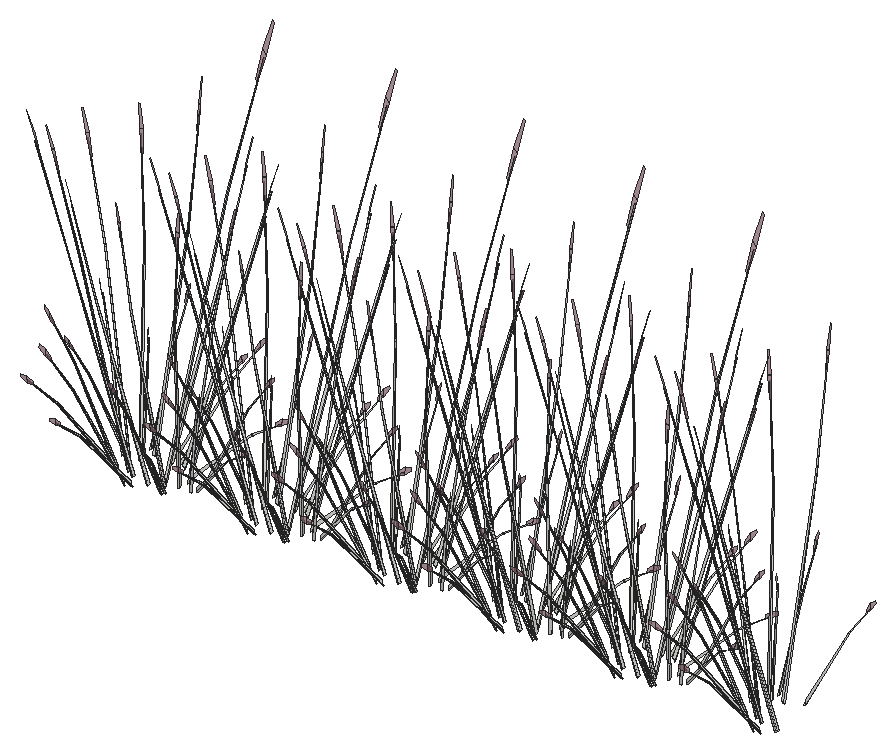
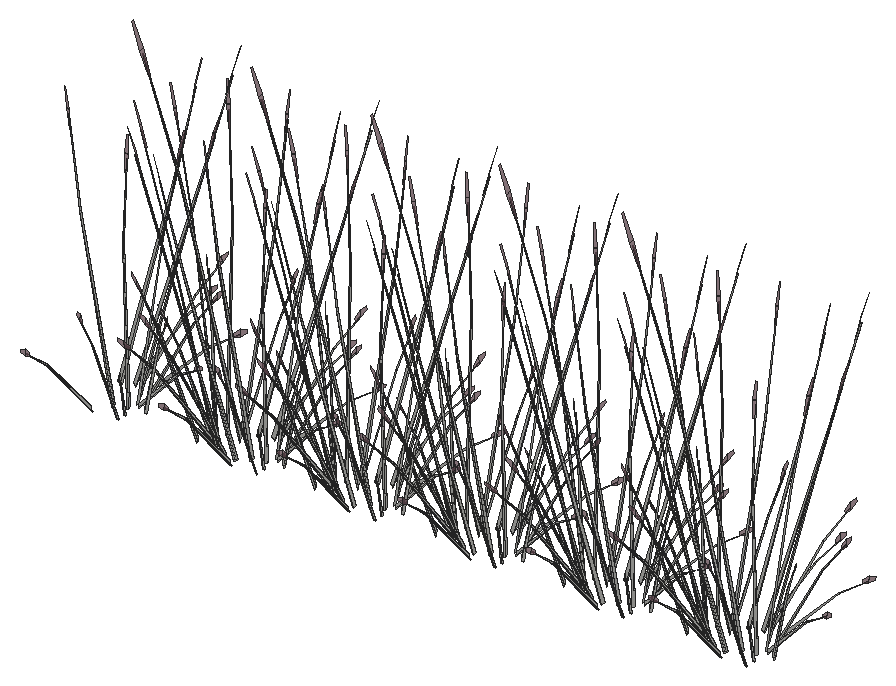
# SketchUp Ruby script. Lengths in inches.
U = 1.inch
M = Sketchup.active_model
def pt(a) = Geom::Point3d.new(a.map { |v| v * U })
def face(e, loops, mat)
  f = e.add_face(loops[0].map { |a| pt(a) })
  loops[1..].each { |l| e.add_face(l.map { |a| pt(a) }).erase! }
  f.material = f.back_material = mat if mat
  f
end
# faces: each face lists its corners as indices into pts; further lists are holes
def faces(e, pts, list, mat = nil) = list.each { |f| face(e, (f[0].is_a?(Array) ? f : [f]).map { |l| l.map { |i| pts[i] } }, mat) }
# xy, xz, yz: faces in a plane at the given z, y or x. An outline is a flat list of corners, or four numbers for a rectangle; further outlines are holes
def ring(l) = l.size == 4 ? [[l[0], l[1]], [l[2], l[1]], [l[2], l[3]], [l[0], l[3]]] : l.each_slice(2).to_a
def flat(e, list, mat, &to3) = list.each { |f| face(e, (f[0].is_a?(Array) ? f : [f]).map { |l| ring(l).map { |u, v| to3.(u, v) } }, mat) }
def xy(e, z, list, mat = nil) = flat(e, list, mat) { |x, y| [x, y, z] }
def xz(e, y, list, mat = nil) = flat(e, list, mat) { |x, z| [x, y, z] }
def yz(e, x, list, mat = nil) = flat(e, list, mat) { |y, z| [x, y, z] }
def lines(e, pts, list) = list.each { |a, b| e.add_line(pt(pts[a]), pt(pts[b])) }
# prism: a flat outline (further loops are holes) pulled along v
def prism(e, loops, v, mat = nil)
  f = face(e, loops, mat); d = Geom::Vector3d.new(v.map { |x| x * U })
  f.pushpull(f.normal.samedirection?(d) ? d.length : -d.length)
end
def box(e, o, s, mat = nil) = prism(e, [[o, [o[0] + s[0], o[1], o[2]], [o[0] + s[0], o[1] + s[1], o[2]], [o[0], o[1] + s[1], o[2]]]], [0, 0, s[2]], mat)
def at(x, y, z, deg = 0) = Geom::Transformation.translation(pt([x, y, z])) * Geom::Transformation.rotation(ORIGIN, Z_AXIS, deg.degrees)
def axes(o, x, y, z) = Geom::Transformation.new([*x, 0, *y, 0, *z, 0, *pt(o).to_a, 1])
def part(name) = M.definitions.add(name)
# library, detail: a bought-in or finely detailed component or shape, given as its bounding box
def library(name, o, s) = part(name).tap { |d| box(d.entities, o, s) }
def detail(e, o, s) = box(e.add_group.entities, o, s)
def put(e, d, t, mat = nil) = e.add_instance(d, t).tap { |i| i.material = mat if mat }
def group(e, t, mat = nil) = e.add_group.tap { |g| g.transformation = t; g.material = mat if mat }.entities
root = M.entities
M.materials.add("LightPink_Translucent").color = [144, 107, 117]
M.materials["LightPink_Translucent"].alpha = 0.75
c1 = part("blade")
p = [[2.15,0.21,22],[0,0.17,0],[0.09,0.45,0],[2.18,0.31,22],[2.29,0.31,22],[0.38,0.45,0],
  [2.48,0.24,33],[2.49,0.24,33],[2.48,0.22,33]]
faces(c1.entities,p,[[0,1,2,3],[4,5,2,3],[6,3,4,7],[8,0,3,6]])
c2 = part("seeds")
p = [[0.3,-0.1,1.38],[-0.01,-0.03,1.59],[-0.01,-0.03,0.03],[0.14,-0.07,-0.07],[0.29,-0.03,3],[0.15,0.01,3.11]]
faces(c2.entities,p,[[0,1,2,3],[1,0,4,5]],"LightPink_Translucent")
c3 = part("blade with seeds")
put(c3.entities,c1,at(0,0,0))
put(c3.entities,c2,axes([2.4,0.25,30.99],[1.5799,-0.05474,1.17369],[-0.12525,1.92788,0.29478],[-0.07173,-0.02425,1.56792]))
put(root,c3,axes([241.68,53.5625,259.72],[-0.12407,0.07933,1.74944],[0.01055,0.57963,-0.27667],[-0.2844,0.07538,0.14031]))
put(root,c3,axes([240.3,54.15,259.71],[0.09697,0.01639,1.77383],[0.29997,0.53988,-0.16761],[-0.1985,0.1417,0.31391]))
put(root,c3,axes([242.27,51.15,259.71],[0.05633,0.06098,1.77383],[-0.27155,0.54815,-0.16761],[-0.27501,0.00397,0.31391]))
put(root,c3,axes([242.9,50.78,259.72],[-0.16348,-0.00431,1.74944],[-0.52047,0.43131,-0.27667],[-0.2777,-0.08813,0.14031]))
put(root,c3,axes([242.48,53.01,260.03],[0.38229,0.5533,-0.1216],[-0.6785,0.2719,-0.67495],[-0.28593,0.073,1.02557]))
put(root,c3,axes([243.34,51.86,260.03],[-0.04068,0.62141,-0.1216],[-0.77029,-0.01698,-0.67495],[-0.29667,-0.04317,1.02557]))
put(root,c3,axes([241.7,55.73,259.72],[-0.01889,0.12092,1.74944],[0.53598,0.42065,-0.27667],[-0.14032,0.19892,0.14031]))
put(root,c3,axes([244.84,50.95,260.43],[-0.50709,0.58578,-0.13619],[-0.73436,-0.33748,-0.75594],[-0.25527,-0.1655,1.14864]))
put(root,c3,axes([242.51,54.33,260.03],[0.70283,0.33692,-0.1216],[-0.40491,0.48793,-0.67495],[-0.19857,0.16961,1.02557]))
put(root,c3,axes([244.65,49.56,259.71],[-0.01417,0.07324,1.77383],[-0.6991,0.2658,-0.16761],[-0.20573,-0.13587,0.31391]))
put(root,c3,axes([241.64,56.97,259.71],[0.0862,-0.03689,1.77383],[0.71245,0.24539,-0.16761],[-0.01674,0.20431,0.31391]))
put(root,c3,axes([245.44,49.84,259.72],[-0.11621,-0.08567,1.74944],[-0.77555,0.05431,-0.27667],[-0.12378,-0.20491,0.14031]))
put(root,c3,axes([243.42,55.45,260.4],[0.83505,0.03027,-0.13498],[-0.02282,0.57322,-0.74919],[-0.05801,0.22077,1.13838]))
put(root,c3,axes([246.62,51.16,260.03],[-0.74352,0.28449,-0.1216],[-0.36538,-0.50492,-0.67495],[-0.0981,-0.21277,1.02557]))
put(root,c3,axes([244.79,57.22,259.72],[0.09631,0.0984,1.74944],[0.77725,0.03866,-0.27667],[0.07816,0.217,0.14031]))
put(root,c3,axes([244.96,56.09,260.03],[0.74352,-0.28449,-0.1216],[0.36538,0.50492,-0.67495],[0.0981,0.21277,1.02557]))
put(root,c3,axes([248.76,50.45,259.71],[-0.07716,0.04667,1.77383],[-0.75601,-0.15746,-0.16761],[-0.02737,-0.20368,0.31391]))
put(root,c3,axes([248.17,51.8,260.03],[-0.83505,-0.03027,-0.1216],[0.02282,-0.57322,-0.67495],[0.05801,-0.22077,1.02557]))
put(root,c3,axes([247.24,52.99,259.47],[-0.65655,-0.31748,1.38283],[0.69326,-0.49431,0.59665],[0.21183,0.29789,1.33663]))
put(root,c3,axes([246.14,56.51,259.71],[0.00225,-0.07398,1.77383],[0.65113,-0.32638,-0.16761],[0.22617,0.1165,0.31391]))
put(root,c3,axes([248.93,50.89,259.72],[-0.00733,-0.12161,1.74944],[-0.61946,-0.35147,-0.27667],[0.09577,-0.21306,0.14031]))
put(root,c3,axes([246.73,56.07,260.03],[0.45276,-0.52302,-0.1216],[0.65568,0.30132,-0.67495],[0.22792,0.14777,1.02557]))
put(root,c3,axes([249.08,52.93,260.03],[-0.70283,-0.33692,-0.1216],[0.40491,-0.48793,-0.67495],[0.19857,-0.16961,1.02557]))
put(root,c3,axes([257.75,53.5625,259.72],[-0.12407,0.07933,1.74944],[0.01055,0.57963,-0.27667],[-0.2844,0.07538,0.14031]))
put(root,c3,axes([256.37,54.15,259.71],[0.09697,0.01639,1.77383],[0.29997,0.53988,-0.16761],[-0.1985,0.1417,0.31391]))
put(root,c3,axes([258.34,51.15,259.71],[0.05633,0.06098,1.77383],[-0.27155,0.54815,-0.16761],[-0.27501,0.00397,0.31391]))
put(root,c3,axes([250.81,52.78,259.71],[-0.09924,-0.00464,1.77383],[-0.4121,-0.49725,-0.16761],[0.1655,-0.1635,0.31391]))
put(root,c3,axes([258.96,50.78,259.72],[-0.16348,-0.00431,1.74944],[-0.52047,0.43131,-0.27667],[-0.2777,-0.08813,0.14031]))
put(root,c3,axes([258.55,53.01,260.03],[0.38229,0.5533,-0.1216],[-0.6785,0.2719,-0.67495],[-0.28593,0.073,1.02557]))
put(root,c3,axes([259.4,51.86,260.03],[-0.04068,0.62141,-0.1216],[-0.77029,-0.01698,-0.67495],[-0.29667,-0.04317,1.02557]))
put(root,c3,axes([248.25,55.4,260.03],[0.04068,-0.62141,-0.1216],[0.77029,0.01698,-0.67495],[0.29667,0.04317,1.02557]))
put(root,c3,axes([249.1,54.25,260.03],[-0.38229,-0.5533,-0.1216],[0.6785,-0.2719,-0.67495],[0.28593,-0.073,1.02557]))
put(root,c3,axes([248.92,55.02,259.72],[0.16299,-0.01033,1.74944],[0.44707,-0.47471,-0.27667],[0.28992,0.06266,0.14031]))
put(root,c3,axes([257.77,55.73,259.72],[-0.01889,0.12092,1.74944],[0.53598,0.42065,-0.27667],[-0.14032,0.19892,0.14031]))
put(root,c3,axes([260.91,50.95,260.43],[-0.50709,0.58578,-0.13619],[-0.73436,-0.33748,-0.75594],[-0.25527,-0.1655,1.14864]))
put(root,c3,axes([250.625,55.89,259.71],[-0.0687,-0.05349,1.77383],[0.15029,-0.57341,-0.16761],[0.27062,-0.03664,0.31391]))
put(root,c3,axes([258.57,54.33,260.03],[0.70283,0.33692,-0.1216],[-0.40491,0.48793,-0.67495],[-0.19857,0.16961,1.02557]))
put(root,c3,axes([251.18,53.38,259.72],[0.10543,-0.09307,1.74944],[-0.13495,-0.57092,-0.27667],[0.26455,-0.10825,0.14031]))
put(root,c3,axes([260.71,49.56,259.71],[-0.01417,0.07324,1.77383],[-0.6991,0.2658,-0.16761],[-0.20573,-0.13587,0.31391]))
put(root,c3,axes([257.71,56.97,259.71],[0.0862,-0.03689,1.77383],[0.71245,0.24539,-0.16761],[-0.01674,0.20431,0.31391]))
put(root,c3,axes([261.51,49.84,259.72],[-0.11621,-0.08567,1.74944],[-0.77555,0.05431,-0.27667],[-0.12378,-0.20491,0.14031]))
put(root,c3,axes([259.48,55.45,260.4],[0.83505,0.03027,-0.13498],[-0.02282,0.57322,-0.74919],[-0.05801,0.22077,1.13838]))
put(root,c3,axes([262.6875,51.16,260.03],[-0.74352,0.28449,-0.1216],[-0.36538,-0.50492,-0.67495],[-0.0981,-0.21277,1.02557]))
put(root,c3,axes([260.85,57.22,259.72],[0.09631,0.0984,1.74944],[0.77725,0.03866,-0.27667],[0.07816,0.217,0.14031]))
put(root,c3,axes([261.03,56.09,260.03],[0.74352,-0.28449,-0.1216],[0.36538,0.50492,-0.67495],[0.0981,0.21277,1.02557]))
put(root,c3,axes([264.83,50.45,259.71],[-0.07716,0.04667,1.77383],[-0.75601,-0.15746,-0.16761],[-0.02737,-0.20368,0.31391]))
put(root,c3,axes([264.23,51.8,260.03],[-0.83505,-0.03027,-0.1216],[0.02282,-0.57322,-0.67495],[0.05801,-0.22077,1.02557]))
put(root,c3,axes([263.31,52.99,259.47],[-0.65655,-0.31748,1.38283],[0.69326,-0.49431,0.59665],[0.21183,0.29789,1.33663]))
put(root,c3,axes([262.2,56.51,259.71],[0.00225,-0.07398,1.77383],[0.65113,-0.32638,-0.16761],[0.22617,0.1165,0.31391]))
put(root,c3,axes([264.99,50.89,259.72],[-0.00733,-0.12161,1.74944],[-0.61946,-0.35147,-0.27667],[0.09577,-0.21306,0.14031]))
put(root,c3,axes([262.79,56.07,260.03],[0.45276,-0.52302,-0.1216],[0.65568,0.30132,-0.67495],[0.22792,0.14777,1.02557]))
put(root,c3,axes([265.14,52.93,260.03],[-0.70283,-0.33692,-0.1216],[0.40491,-0.48793,-0.67495],[0.19857,-0.16961,1.02557]))
put(root,c3,axes([274.48,53.5625,259.72],[-0.12407,0.07933,1.74944],[0.01055,0.57963,-0.27667],[-0.2844,0.07538,0.14031]))
put(root,c3,axes([266.87,52.78,259.71],[-0.09924,-0.00464,1.77383],[-0.4121,-0.49725,-0.16761],[0.1655,-0.1635,0.31391]))
put(root,c3,axes([273.1,54.15,259.71],[0.09697,0.01639,1.77383],[0.29997,0.53988,-0.16761],[-0.1985,0.1417,0.31391]))
put(root,c3,axes([264.3125,55.4,260.03],[0.04068,-0.62141,-0.1216],[0.77029,0.01698,-0.67495],[0.29667,0.04317,1.02557]))
put(root,c3,axes([265.17,54.25,260.03],[-0.38229,-0.5533,-0.1216],[0.6785,-0.2719,-0.67495],[0.28593,-0.073,1.02557]))
put(root,c3,axes([275.0625,51.15,259.71],[0.05633,0.06098,1.77383],[-0.27155,0.54815,-0.16761],[-0.27501,0.00397,0.31391]))
put(root,c3,axes([275.69,50.78,259.72],[-0.16348,-0.00431,1.74944],[-0.52047,0.43131,-0.27667],[-0.2777,-0.08813,0.14031]))
put(root,c3,axes([275.27,53.01,260.03],[0.38229,0.5533,-0.1216],[-0.6785,0.2719,-0.67495],[-0.28593,0.073,1.02557]))
put(root,c3,axes([276.13,51.86,260.03],[-0.04068,0.62141,-0.1216],[-0.77029,-0.01698,-0.67495],[-0.29667,-0.04317,1.02557]))
put(root,c3,axes([264.98,55.02,259.72],[0.16299,-0.01033,1.74944],[0.44707,-0.47471,-0.27667],[0.28992,0.06266,0.14031]))
put(root,c3,axes([266.69,55.89,259.71],[-0.0687,-0.05349,1.77383],[0.15029,-0.57341,-0.16761],[0.27062,-0.03664,0.31391]))
put(root,c3,axes([274.5,55.73,259.72],[-0.01889,0.12092,1.74944],[0.53598,0.42065,-0.27667],[-0.14032,0.19892,0.14031]))
put(root,c3,axes([277.64,50.95,260.43],[-0.50709,0.58578,-0.13619],[-0.73436,-0.33748,-0.75594],[-0.25527,-0.1655,1.14864]))
put(root,c3,axes([267.25,53.38,259.72],[0.10543,-0.09307,1.74944],[-0.13495,-0.57092,-0.27667],[0.26455,-0.10825,0.14031]))
put(root,c3,axes([275.3,54.33,260.03],[0.70283,0.33692,-0.1216],[-0.40491,0.48793,-0.67495],[-0.19857,0.16961,1.02557]))
put(root,c3,axes([277.44,49.56,259.71],[-0.01417,0.07324,1.77383],[-0.6991,0.2658,-0.16761],[-0.20573,-0.13587,0.31391]))
put(root,c3,axes([274.4375,56.97,259.71],[0.0862,-0.03689,1.77383],[0.71245,0.24539,-0.16761],[-0.01674,0.20431,0.31391]))
put(root,c3,axes([278.24,49.84,259.72],[-0.11621,-0.08567,1.74944],[-0.77555,0.05431,-0.27667],[-0.12378,-0.20491,0.14031]))
put(root,c3,axes([276.21,55.45,260.4],[0.83505,0.03027,-0.13498],[-0.02282,0.57322,-0.74919],[-0.05801,0.22077,1.13838]))
put(root,c3,axes([279.42,51.16,260.03],[-0.74352,0.28449,-0.1216],[-0.36538,-0.50492,-0.67495],[-0.0981,-0.21277,1.02557]))
put(root,c3,axes([277.58,57.22,259.72],[0.09631,0.0984,1.74944],[0.77725,0.03866,-0.27667],[0.07816,0.217,0.14031]))
put(root,c3,axes([277.76,56.09,260.03],[0.74352,-0.28449,-0.1216],[0.36538,0.50492,-0.67495],[0.0981,0.21277,1.02557]))
put(root,c3,axes([281.55,50.45,259.71],[-0.07716,0.04667,1.77383],[-0.75601,-0.15746,-0.16761],[-0.02737,-0.20368,0.31391]))
put(root,c3,axes([280.96,51.8,260.03],[-0.83505,-0.03027,-0.1216],[0.02282,-0.57322,-0.67495],[0.05801,-0.22077,1.02557]))
put(root,c3,axes([280.04,52.99,259.47],[-0.65655,-0.31748,1.38283],[0.69326,-0.49431,0.59665],[0.21183,0.29789,1.33663]))
put(root,c3,axes([278.93,56.51,259.71],[0.00225,-0.07398,1.77383],[0.65113,-0.32638,-0.16761],[0.22617,0.1165,0.31391]))
put(root,c3,axes([281.72,50.89,259.72],[-0.00733,-0.12161,1.74944],[-0.61946,-0.35147,-0.27667],[0.09577,-0.21306,0.14031]))
put(root,c3,axes([279.52,56.07,260.03],[0.45276,-0.52302,-0.1216],[0.65568,0.30132,-0.67495],[0.22792,0.14777,1.02557]))
put(root,c3,axes([281.87,52.93,260.03],[-0.70283,-0.33692,-0.1216],[0.40491,-0.48793,-0.67495],[0.19857,-0.16961,1.02557]))
put(root,c3,axes([290.2,53.5625,259.72],[-0.12407,0.07933,1.74944],[0.01055,0.57963,-0.27667],[-0.2844,0.07538,0.14031]))
put(root,c3,axes([288.83,54.15,259.71],[0.09697,0.01639,1.77383],[0.29997,0.53988,-0.16761],[-0.1985,0.1417,0.31391]))
put(root,c3,axes([290.79,51.15,259.71],[0.05633,0.06098,1.77383],[-0.27155,0.54815,-0.16761],[-0.27501,0.00397,0.31391]))
put(root,c3,axes([291.42,50.78,259.72],[-0.16348,-0.00431,1.74944],[-0.52047,0.43131,-0.27667],[-0.2777,-0.08813,0.14031]))
put(root,c3,axes([291,53.01,260.03],[0.38229,0.5533,-0.1216],[-0.6785,0.2719,-0.67495],[-0.28593,0.073,1.02557]))
put(root,c3,axes([291.86,51.86,260.03],[-0.04068,0.62141,-0.1216],[-0.77029,-0.01698,-0.67495],[-0.29667,-0.04317,1.02557]))
put(root,c3,axes([283.6,52.78,259.71],[-0.09924,-0.00464,1.77383],[-0.4121,-0.49725,-0.16761],[0.1655,-0.1635,0.31391]))
put(root,c3,axes([281.04,55.4,260.03],[0.04068,-0.62141,-0.1216],[0.77029,0.01698,-0.67495],[0.29667,0.04317,1.02557]))
put(root,c3,axes([281.9,54.25,260.03],[-0.38229,-0.5533,-0.1216],[0.6785,-0.2719,-0.67495],[0.28593,-0.073,1.02557]))
put(root,c3,axes([281.71,55.02,259.72],[0.16299,-0.01033,1.74944],[0.44707,-0.47471,-0.27667],[0.28992,0.06266,0.14031]))
put(root,c3,axes([290.23,55.73,259.72],[-0.01889,0.12092,1.74944],[0.53598,0.42065,-0.27667],[-0.14032,0.19892,0.14031]))
put(root,c3,axes([293.37,50.95,260.43],[-0.50709,0.58578,-0.13619],[-0.73436,-0.33748,-0.75594],[-0.25527,-0.1655,1.14864]))
put(root,c3,axes([283.42,55.89,259.71],[-0.0687,-0.05349,1.77383],[0.15029,-0.57341,-0.16761],[0.27062,-0.03664,0.31391]))
put(root,c3,axes([291.03,54.33,260.03],[0.70283,0.33692,-0.1216],[-0.40491,0.48793,-0.67495],[-0.19857,0.16961,1.02557]))
put(root,c3,axes([283.97,53.38,259.72],[0.10543,-0.09307,1.74944],[-0.13495,-0.57092,-0.27667],[0.26455,-0.10825,0.14031]))
put(root,c3,axes([293.17,49.56,259.71],[-0.01417,0.07324,1.77383],[-0.6991,0.2658,-0.16761],[-0.20573,-0.13587,0.31391]))
put(root,c3,axes([290.16,56.97,259.71],[0.0862,-0.03689,1.77383],[0.71245,0.24539,-0.16761],[-0.01674,0.20431,0.31391]))
put(root,c3,axes([293.96,49.84,259.72],[-0.11621,-0.08567,1.74944],[-0.77555,0.05431,-0.27667],[-0.12378,-0.20491,0.14031]))
put(root,c3,axes([291.9375,55.45,260.4],[0.83505,0.03027,-0.13498],[-0.02282,0.57322,-0.74919],[-0.05801,0.22077,1.13838]))
put(root,c3,axes([295.14,51.16,260.03],[-0.74352,0.28449,-0.1216],[-0.36538,-0.50492,-0.67495],[-0.0981,-0.21277,1.02557]))
put(root,c3,axes([293.31,57.22,259.72],[0.09631,0.0984,1.74944],[0.77725,0.03866,-0.27667],[0.07816,0.217,0.14031]))
put(root,c3,axes([293.48,56.09,260.03],[0.74352,-0.28449,-0.1216],[0.36538,0.50492,-0.67495],[0.0981,0.21277,1.02557]))
put(root,c3,axes([297.28,50.45,259.71],[-0.07716,0.04667,1.77383],[-0.75601,-0.15746,-0.16761],[-0.02737,-0.20368,0.31391]))
put(root,c3,axes([296.6875,51.8,260.03],[-0.83505,-0.03027,-0.1216],[0.02282,-0.57322,-0.67495],[0.05801,-0.22077,1.02557]))
put(root,c3,axes([295.76,52.99,259.47],[-0.65655,-0.31748,1.38283],[0.69326,-0.49431,0.59665],[0.21183,0.29789,1.33663]))
put(root,c3,axes([294.66,56.51,259.71],[0.00225,-0.07398,1.77383],[0.65113,-0.32638,-0.16761],[0.22617,0.1165,0.31391]))
put(root,c3,axes([297.45,50.89,259.72],[-0.00733,-0.12161,1.74944],[-0.61946,-0.35147,-0.27667],[0.09577,-0.21306,0.14031]))
put(root,c3,axes([295.25,56.07,260.03],[0.45276,-0.52302,-0.1216],[0.65568,0.30132,-0.67495],[0.22792,0.14777,1.02557]))
put(root,c3,axes([297.6,52.93,260.03],[-0.70283,-0.33692,-0.1216],[0.40491,-0.48793,-0.67495],[0.19857,-0.16961,1.02557]))
put(root,c3,axes([305.65,53.5625,259.72],[-0.12407,0.07933,1.74944],[0.01055,0.57963,-0.27667],[-0.2844,0.07538,0.14031]))
put(root,c3,axes([304.27,54.15,259.71],[0.09697,0.01639,1.77383],[0.29997,0.53988,-0.16761],[-0.1985,0.1417,0.31391]))
put(root,c3,axes([306.24,51.15,259.71],[0.05633,0.06098,1.77383],[-0.27155,0.54815,-0.16761],[-0.27501,0.00397,0.31391]))
put(root,c3,axes([306.87,50.78,259.72],[-0.16348,-0.00431,1.74944],[-0.52047,0.43131,-0.27667],[-0.2777,-0.08813,0.14031]))
put(root,c3,axes([306.45,53.01,260.03],[0.38229,0.5533,-0.1216],[-0.6785,0.2719,-0.67495],[-0.28593,0.073,1.02557]))
put(root,c3,axes([307.31,51.86,260.03],[-0.04068,0.62141,-0.1216],[-0.77029,-0.01698,-0.67495],[-0.29667,-0.04317,1.02557]))
put(root,c3,axes([299.33,52.78,259.71],[-0.09924,-0.00464,1.77383],[-0.4121,-0.49725,-0.16761],[0.1655,-0.1635,0.31391]))
put(root,c3,axes([296.77,55.4,260.03],[0.04068,-0.62141,-0.1216],[0.77029,0.01698,-0.67495],[0.29667,0.04317,1.02557]))
put(root,c3,axes([297.625,54.25,260.03],[-0.38229,-0.5533,-0.1216],[0.6785,-0.2719,-0.67495],[0.28593,-0.073,1.02557]))
put(root,c3,axes([297.4375,55.02,259.72],[0.16299,-0.01033,1.74944],[0.44707,-0.47471,-0.27667],[0.28992,0.06266,0.14031]))
put(root,c3,axes([305.67,55.73,259.72],[-0.01889,0.12092,1.74944],[0.53598,0.42065,-0.27667],[-0.14032,0.19892,0.14031]))
put(root,c3,axes([308.8125,50.95,260.43],[-0.50709,0.58578,-0.13619],[-0.73436,-0.33748,-0.75594],[-0.25527,-0.1655,1.14864]))
put(root,c3,axes([306.48,54.33,260.03],[0.70283,0.33692,-0.1216],[-0.40491,0.48793,-0.67495],[-0.19857,0.16961,1.02557]))
put(root,c3,axes([299.15,55.89,259.71],[-0.0687,-0.05349,1.77383],[0.15029,-0.57341,-0.16761],[0.27062,-0.03664,0.31391]))
put(root,c3,axes([299.7,53.38,259.72],[0.10543,-0.09307,1.74944],[-0.13495,-0.57092,-0.27667],[0.26455,-0.10825,0.14031]))
put(root,c3,axes([308.62,49.56,259.71],[-0.01417,0.07324,1.77383],[-0.6991,0.2658,-0.16761],[-0.20573,-0.13587,0.31391]))
put(root,c3,axes([305.61,56.97,259.71],[0.0862,-0.03689,1.77383],[0.71245,0.24539,-0.16761],[-0.01674,0.20431,0.31391]))
put(root,c3,axes([309.41,49.84,259.72],[-0.11621,-0.08567,1.74944],[-0.77555,0.05431,-0.27667],[-0.12378,-0.20491,0.14031]))
put(root,c3,axes([307.39,55.45,260.4],[0.83505,0.03027,-0.13498],[-0.02282,0.57322,-0.74919],[-0.05801,0.22077,1.13838]))
put(root,c3,axes([310.59,51.16,260.03],[-0.74352,0.28449,-0.1216],[-0.36538,-0.50492,-0.67495],[-0.0981,-0.21277,1.02557]))
put(root,c3,axes([308.76,57.22,259.72],[0.09631,0.0984,1.74944],[0.77725,0.03866,-0.27667],[0.07816,0.217,0.14031]))
put(root,c3,axes([308.93,56.09,260.03],[0.74352,-0.28449,-0.1216],[0.36538,0.50492,-0.67495],[0.0981,0.21277,1.02557]))
put(root,c3,axes([312.73,50.45,259.71],[-0.07716,0.04667,1.77383],[-0.75601,-0.15746,-0.16761],[-0.02737,-0.20368,0.31391]))
put(root,c3,axes([312.14,51.8,260.03],[-0.83505,-0.03027,-0.1216],[0.02282,-0.57322,-0.67495],[0.05801,-0.22077,1.02557]))
put(root,c3,axes([311.21,52.99,259.47],[-0.65655,-0.31748,1.38283],[0.69326,-0.49431,0.59665],[0.21183,0.29789,1.33663]))
put(root,c3,axes([310.11,56.51,259.71],[0.00225,-0.07398,1.77383],[0.65113,-0.32638,-0.16761],[0.22617,0.1165,0.31391]))
put(root,c3,axes([312.9,50.89,259.72],[-0.00733,-0.12161,1.74944],[-0.61946,-0.35147,-0.27667],[0.09577,-0.21306,0.14031]))
put(root,c3,axes([310.7,56.07,260.03],[0.45276,-0.52302,-0.1216],[0.65568,0.30132,-0.67495],[0.22792,0.14777,1.02557]))
put(root,c3,axes([313.05,52.93,260.03],[-0.70283,-0.33692,-0.1216],[0.40491,-0.48793,-0.67495],[0.19857,-0.16961,1.02557]))
put(root,c3,axes([314.78,52.78,259.71],[-0.09924,-0.00464,1.77383],[-0.4121,-0.49725,-0.16761],[0.1655,-0.1635,0.31391]))
put(root,c3,axes([312.22,55.4,260.03],[0.04068,-0.62141,-0.1216],[0.77029,0.01698,-0.67495],[0.29667,0.04317,1.02557]))
put(root,c3,axes([313.07,54.25,260.03],[-0.38229,-0.5533,-0.1216],[0.6785,-0.2719,-0.67495],[0.28593,-0.073,1.02557]))
put(root,c3,axes([323.76,53.5625,259.72],[-0.12407,0.07933,1.74944],[0.01055,0.57963,-0.27667],[-0.2844,0.07538,0.14031]))
put(root,c3,axes([312.89,55.02,259.72],[0.16299,-0.01033,1.74944],[0.44707,-0.47471,-0.27667],[0.28992,0.06266,0.14031]))
put(root,c3,axes([322.38,54.15,259.71],[0.09697,0.01639,1.77383],[0.29997,0.53988,-0.16761],[-0.1985,0.1417,0.31391]))
put(root,c3,axes([324.35,51.15,259.71],[0.05633,0.06098,1.77383],[-0.27155,0.54815,-0.16761],[-0.27501,0.00397,0.31391]))
put(root,c3,axes([314.59,55.89,259.71],[-0.0687,-0.05349,1.77383],[0.15029,-0.57341,-0.16761],[0.27062,-0.03664,0.31391]))
put(root,c3,axes([324.98,50.78,259.72],[-0.16348,-0.00431,1.74944],[-0.52047,0.43131,-0.27667],[-0.2777,-0.08813,0.14031]))
put(root,c3,axes([324.56,53.01,260.03],[0.38229,0.5533,-0.1216],[-0.6785,0.2719,-0.67495],[-0.28593,0.073,1.02557]))
put(root,c3,axes([325.42,51.86,260.03],[-0.04068,0.62141,-0.1216],[-0.77029,-0.01698,-0.67495],[-0.29667,-0.04317,1.02557]))
put(root,c3,axes([315.15,53.38,259.72],[0.10543,-0.09307,1.74944],[-0.13495,-0.57092,-0.27667],[0.26455,-0.10825,0.14031]))
put(root,c3,axes([323.78,55.73,259.72],[-0.01889,0.12092,1.74944],[0.53598,0.42065,-0.27667],[-0.14032,0.19892,0.14031]))
put(root,c3,axes([326.92,50.95,260.43],[-0.50709,0.58578,-0.13619],[-0.73436,-0.33748,-0.75594],[-0.25527,-0.1655,1.14864]))
put(root,c3,axes([324.59,54.33,260.03],[0.70283,0.33692,-0.1216],[-0.40491,0.48793,-0.67495],[-0.19857,0.16961,1.02557]))
put(root,c3,axes([326.72,49.56,259.71],[-0.01417,0.07324,1.77383],[-0.6991,0.2658,-0.16761],[-0.20573,-0.13587,0.31391]))
put(root,c3,axes([323.72,56.97,259.71],[0.0862,-0.03689,1.77383],[0.71245,0.24539,-0.16761],[-0.01674,0.20431,0.31391]))
put(root,c3,axes([327.52,49.84,259.72],[-0.11621,-0.08567,1.74944],[-0.77555,0.05431,-0.27667],[-0.12378,-0.20491,0.14031]))
put(root,c3,axes([325.49,55.45,260.4],[0.83505,0.03027,-0.13498],[-0.02282,0.57322,-0.74919],[-0.05801,0.22077,1.13838]))
put(root,c3,axes([328.7,51.16,260.03],[-0.74352,0.28449,-0.1216],[-0.36538,-0.50492,-0.67495],[-0.0981,-0.21277,1.02557]))
put(root,c3,axes([326.86,57.22,259.72],[0.09631,0.0984,1.74944],[0.77725,0.03866,-0.27667],[0.07816,0.217,0.14031]))
